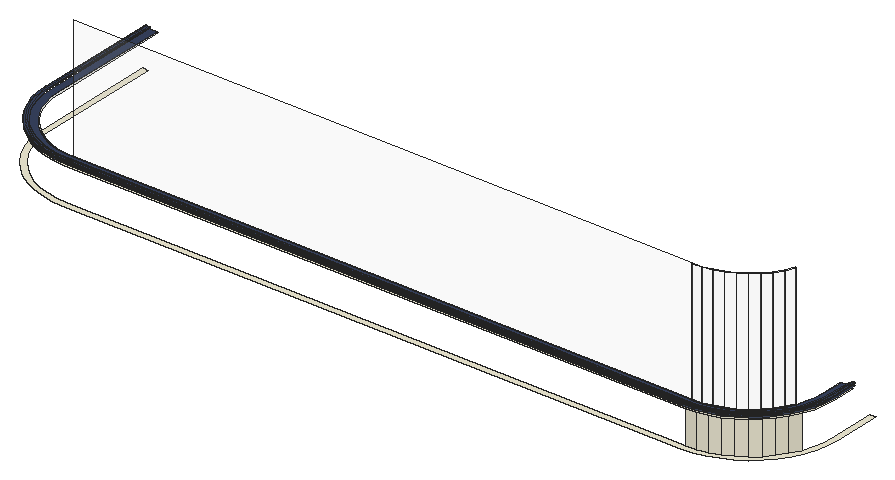
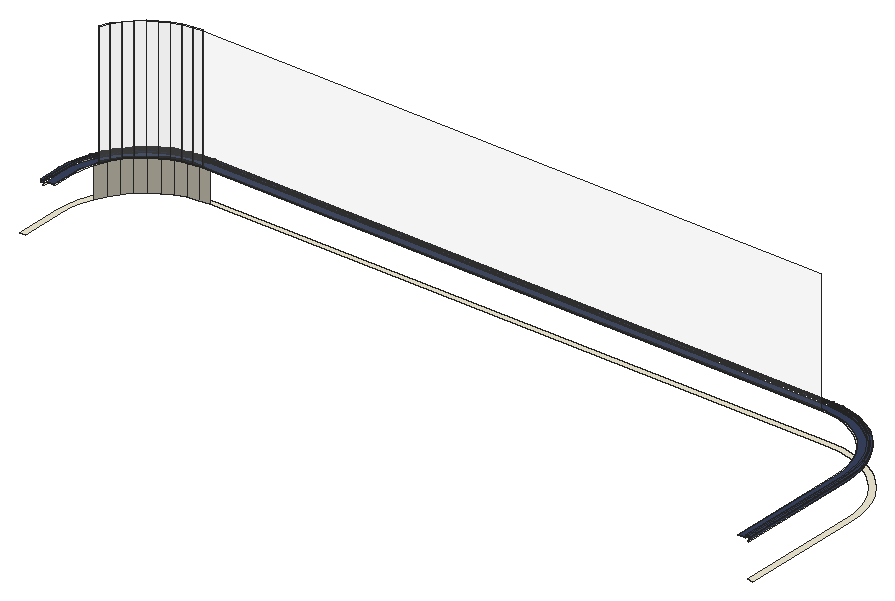
# SketchUp Ruby script. Lengths in inches.
U = 1.inch
M = Sketchup.active_model
def pt(a) = Geom::Point3d.new(a.map { |v| v * U })
def face(e, loops, mat)
  f = e.add_face(loops[0].map { |a| pt(a) })
  loops[1..].each { |l| e.add_face(l.map { |a| pt(a) }).erase! }
  f.material = f.back_material = mat if mat
  f
end
# faces: each face lists its corners as indices into pts; further lists are holes
def faces(e, pts, list, mat = nil) = list.each { |f| face(e, (f[0].is_a?(Array) ? f : [f]).map { |l| l.map { |i| pts[i] } }, mat) }
# xy, xz, yz: faces in a plane at the given z, y or x. An outline is a flat list of corners, or four numbers for a rectangle; further outlines are holes
def ring(l) = l.size == 4 ? [[l[0], l[1]], [l[2], l[1]], [l[2], l[3]], [l[0], l[3]]] : l.each_slice(2).to_a
def flat(e, list, mat, &to3) = list.each { |f| face(e, (f[0].is_a?(Array) ? f : [f]).map { |l| ring(l).map { |u, v| to3.(u, v) } }, mat) }
def xy(e, z, list, mat = nil) = flat(e, list, mat) { |x, y| [x, y, z] }
def xz(e, y, list, mat = nil) = flat(e, list, mat) { |x, z| [x, y, z] }
def yz(e, x, list, mat = nil) = flat(e, list, mat) { |y, z| [x, y, z] }
def lines(e, pts, list) = list.each { |a, b| e.add_line(pt(pts[a]), pt(pts[b])) }
# prism: a flat outline (further loops are holes) pulled along v
def prism(e, loops, v, mat = nil)
  f = face(e, loops, mat); d = Geom::Vector3d.new(v.map { |x| x * U })
  f.pushpull(f.normal.samedirection?(d) ? d.length : -d.length)
end
def box(e, o, s, mat = nil) = prism(e, [[o, [o[0] + s[0], o[1], o[2]], [o[0] + s[0], o[1] + s[1], o[2]], [o[0], o[1] + s[1], o[2]]]], [0, 0, s[2]], mat)
def at(x, y, z, deg = 0) = Geom::Transformation.translation(pt([x, y, z])) * Geom::Transformation.rotation(ORIGIN, Z_AXIS, deg.degrees)
def axes(o, x, y, z) = Geom::Transformation.new([*x, 0, *y, 0, *z, 0, *pt(o).to_a, 1])
def part(name) = M.definitions.add(name)
# library, detail: a bought-in or finely detailed component or shape, given as its bounding box
def library(name, o, s) = part(name).tap { |d| box(d.entities, o, s) }
def detail(e, o, s) = box(e.add_group.entities, o, s)
def put(e, d, t, mat = nil) = e.add_instance(d, t).tap { |i| i.material = mat if mat }
def group(e, t, mat = nil) = e.add_group.tap { |g| g.transformation = t; g.material = mat if mat }.entities
root = M.entities
M.materials.add("0344 AP 9635 Ganges Midnight-N").color = [69, 80, 105]
M.materials.add("0360 AP 9644 Monsoon Midnight-N").color = [56, 67, 95]
M.materials.add("0905 AP 7844 MILD YELLOW").color = [242, 237, 215]
M.materials.add("Glass Clear 001").color = [246, 246, 246]
M.materials["Glass Clear 001"].alpha = 0.1
xy(root,121.25,[[57,28.27,238.5625,28.27,241.91,28.49,245.21,29.14,248.39,30.22,251.4,31.71,254.19,33.57,256.71,35.79,258.93,38.31,260.79,41.1,262.28,44.11,263.36,47.29,264.01,50.59,264.23,53.9375,264.23,67.61,262.5625,67.61,262.5625,53.9375,262.36,50.8,261.74,47.73,260.74,44.75,259.35,41.9375,257.6,39.33,255.53,36.97,253.17,34.9,250.5625,33.15,247.75,31.76,244.77,30.76,241.7,30.14,238.5625,29.9375,57,29.9375,53.87,30.14,50.79,30.76,47.82,31.76,45,33.15,42.39,34.9,40.03,36.97,37.96,39.33,36.22,41.9375,34.83,44.75,33.82,47.73,33.21,50.8,33,53.9375,33,89.9375,31.33,89.9375,31.33,53.9375,31.55,50.59,32.2,47.29,33.28,44.11,34.77,41.1,36.63,38.31,38.85,35.79,41.37,33.57,44.16,31.71,47.18,30.22,50.36,29.14,53.65,28.49]],"0905 AP 7844 MILD YELLOW")
xy(root,131.3125,[[57,29.45,53.8,29.65,50.66,30.28,47.63,31.31,44.75,32.73,42.09,34.51,39.68,36.62,37.57,39.03,35.79,41.69,34.37,44.56,33.34,47.6,32.72,50.74,32.51,53.9375,32.51,89.9375,33,89.9375,33,53.9375,33.21,50.8,33.82,47.73,34.83,44.75,36.22,41.9375,37.96,39.33,40.03,36.97,42.39,34.9,45,33.15,47.82,31.76,50.79,30.76,53.87,30.14,57,29.9375,238.5625,29.9375,241.7,30.14,244.77,30.76,247.75,31.76,250.5625,33.15,253.17,34.9,255.53,36.97,257.6,39.33,259.35,41.9375,260.74,44.75,261.74,47.73,262.36,50.8,262.5625,53.9375,262.5625,60.55,263.05,60.55,263.05,53.9375,262.85,50.74,262.22,47.6,261.19,44.56,259.77,41.69,257.99,39.03,255.88,36.62,253.47,34.51,250.81,32.73,247.94,31.31,244.9,30.28,241.76,29.65,238.5625,29.45]],"0905 AP 7844 MILD YELLOW")
xy(root,132,[[57,32.3125,54.18,32.5,51.4,33.05,48.72,33.96,46.1875,35.21,43.84,36.78,41.71,38.65,39.84,40.77,38.27,43.125,37.02,45.66,36.11,48.34,35.56,51.11,35.375,53.9375,35.375,89.9375,35.75,89.9375,35.75,53.9375,35.94,51.16,36.48,48.4375,37.37,45.81,38.6,43.3125,40.14,41,41.98,38.91,44.07,37.08,46.375,35.54,48.87,34.31,51.5,33.41,54.23,32.87,57,32.69,238.5625,32.69,241.34,32.87,244.0625,33.41,246.69,34.31,249.1875,35.54,251.5,37.08,253.59,38.91,255.42,41,256.96,43.3125,258.19,45.81,259.09,48.4375,259.63,51.16,259.81,53.9375,259.81,60.0625,260.1875,60.0625,260.1875,53.9375,260,51.11,259.45,48.34,258.54,45.66,257.29,43.125,255.72,40.77,253.85,38.65,251.73,36.78,249.375,35.21,246.84,33.96,244.16,33.05,241.39,32.5,238.5625,32.3125]])
xy(root,132,[[57,29.09,53.76,29.31,50.57,29.9375,47.49,30.98,44.58,32.42,41.875,34.23,39.43,36.37,37.29,38.8125,35.48,41.51,34.05,44.43,33,47.51,32.37,50.69,32.15,53.9375,32.15,89.9375,32.51,89.9375,32.51,53.9375,32.72,50.74,33.34,47.6,34.37,44.56,35.79,41.69,37.57,39.03,39.68,36.62,42.09,34.51,44.75,32.73,47.63,31.31,50.66,30.28,53.8,29.65,57,29.45,238.5625,29.45,241.76,29.65,244.9,30.28,247.94,31.31,250.81,32.73,253.47,34.51,255.88,36.62,257.99,39.03,259.77,41.69,261.19,44.56,262.22,47.6,262.85,50.74,263.05,53.9375,263.05,60.55,262.5625,60.55,262.5625,60.91,263.41,60.91,263.41,53.9375,263.19,50.69,262.5625,47.51,261.52,44.43,260.08,41.51,258.27,38.8125,256.13,36.37,253.6875,34.23,250.99,32.42,248.07,30.98,244.99,29.9375,241.81,29.31,238.5625,29.09],[57,30.29,53.91,30.49,50.88,31.1,47.95,32.09,45.18,33.46,42.6,35.18,40.28,37.22,38.24,39.54,36.52,42.11,35.15,44.89,34.16,47.82,33.56,50.85,33.35,53.9375,33.35,89.9375,35.375,89.9375,35.375,53.9375,35.56,51.11,36.11,48.34,37.02,45.66,38.27,43.125,39.84,40.77,41.71,38.65,43.84,36.78,46.1875,35.21,48.72,33.96,51.4,33.05,54.18,32.5,57,32.3125,238.5625,32.3125,241.39,32.5,244.16,33.05,246.84,33.96,249.375,35.21,251.73,36.78,253.85,38.65,255.72,40.77,257.29,43.125,258.54,45.66,259.45,48.34,260,51.11,260.1875,53.9375,260.1875,60.0625,262.21,60.0625,262.21,53.9375,262.01,50.85,261.4,47.82,260.41,44.89,259.04,42.11,257.32,39.54,255.28,37.22,252.96,35.18,250.39,33.46,247.61,32.09,244.68,31.1,241.65,30.49,238.5625,30.29]],"0360 AP 9644 Monsoon Midnight-N")
xy(root,132.1875,[[57,30.29,238.5625,30.29,241.65,30.49,244.68,31.1,247.61,32.09,250.39,33.46,252.96,35.18,255.28,37.22,257.32,39.54,259.04,42.11,260.41,44.89,261.4,47.82,262.01,50.85,262.21,53.9375,262.21,60.0625,260.1875,60.0625,260.1875,53.9375,260,51.11,259.45,48.34,258.54,45.66,257.29,43.125,255.72,40.77,253.85,38.65,251.73,36.78,249.375,35.21,246.84,33.96,244.16,33.05,241.39,32.5,238.5625,32.3125,57,32.3125,54.18,32.5,51.4,33.05,48.72,33.96,46.1875,35.21,43.84,36.78,41.71,38.65,39.84,40.77,38.27,43.125,37.02,45.66,36.11,48.34,35.56,51.11,35.375,53.9375,35.375,89.9375,33.35,89.9375,33.35,53.9375,33.56,50.85,34.16,47.82,35.15,44.89,36.52,42.11,38.24,39.54,40.28,37.22,42.6,35.18,45.18,33.46,47.95,32.09,50.88,31.1,53.91,30.49]],"0360 AP 9644 Monsoon Midnight-N")
xy(root,132.5625,[[57,29.01,53.75,29.23,50.55,29.86,47.46,30.91,44.54,32.35,41.83,34.16,39.375,36.3125,37.23,38.76,35.41,41.47,33.97,44.4,32.92,47.49,32.29,50.68,32.07,53.9375,32.07,90.02,32.59,90.02,32.59,89.9375,32.15,89.9375,32.15,53.9375,32.37,50.69,33,47.51,34.05,44.43,35.48,41.51,37.29,38.8125,39.43,36.37,41.875,34.23,44.58,32.42,47.49,30.98,50.57,29.9375,53.76,29.31,57,29.09,238.5625,29.09,241.81,29.31,244.99,29.9375,248.07,30.98,250.99,32.42,253.6875,34.23,256.13,36.37,258.27,38.8125,260.08,41.51,261.52,44.43,262.5625,47.51,263.19,50.69,263.41,53.9375,263.41,60.91,262.5625,60.91,262.5625,60.47,262.48,60.47,262.48,60.99,263.49,60.99,263.49,53.9375,263.27,50.68,262.64,47.49,261.59,44.4,260.15,41.47,258.34,38.76,256.1875,36.3125,253.74,34.16,251.03,32.35,248.1,30.91,245.01,29.86,241.82,29.23,238.5625,29.01]],"0360 AP 9644 Monsoon Midnight-N")
xy(root,132.625,[[57,29.01,53.75,29.23,50.55,29.86,47.46,30.91,44.54,32.35,41.83,34.16,39.375,36.3125,37.23,38.76,35.41,41.47,33.97,44.4,32.92,47.49,32.29,50.68,32.07,53.9375,32.07,90.02,32.59,90.02,32.59,89.9375,32.15,89.9375,32.15,53.9375,32.37,50.69,33,47.51,34.05,44.43,35.48,41.51,37.29,38.8125,39.43,36.37,41.875,34.23,44.58,32.42,47.49,30.98,50.57,29.9375,53.76,29.31,57,29.09,238.5625,29.09,241.81,29.31,244.99,29.9375,248.07,30.98,250.99,32.42,253.6875,34.23,256.13,36.37,258.27,38.8125,260.08,41.51,261.52,44.43,262.5625,47.51,263.19,50.69,263.41,53.9375,263.41,60.91,262.5625,60.91,262.5625,60.47,262.48,60.47,262.48,60.99,263.49,60.99,263.49,53.9375,263.27,50.68,262.64,47.49,261.59,44.4,260.15,41.47,258.34,38.76,256.1875,36.3125,253.74,34.16,251.03,32.35,248.1,30.91,245.01,29.86,241.82,29.23,238.5625,29.01],[57,29.09,53.76,29.31,50.57,29.9375,47.49,30.98,44.58,32.42,41.875,34.23,39.43,36.37,37.29,38.8125,35.48,41.51,34.05,44.43,33,47.51,32.37,50.69,32.15,53.9375,32.15,89.9375,32.51,89.9375,32.51,53.9375,32.72,50.74,33.34,47.6,34.37,44.56,35.79,41.69,37.57,39.03,39.68,36.62,42.09,34.51,44.75,32.73,47.63,31.31,50.66,30.28,53.8,29.65,57,29.45,238.5625,29.45,241.76,29.65,244.9,30.28,247.94,31.31,250.81,32.73,253.47,34.51,255.88,36.62,257.99,39.03,259.77,41.69,261.19,44.56,262.22,47.6,262.85,50.74,263.05,53.9375,263.05,60.55,262.5625,60.55,262.5625,60.91,263.41,60.91,263.41,53.9375,263.19,50.69,262.5625,47.51,261.52,44.43,260.08,41.51,258.27,38.8125,256.13,36.37,253.6875,34.23,250.99,32.42,248.07,30.98,244.99,29.9375,241.81,29.31,238.5625,29.09],[57,29.45,53.8,29.65,50.66,30.28,47.63,31.31,44.75,32.73,42.09,34.51,39.68,36.62,37.57,39.03,35.79,41.69,34.37,44.56,33.34,47.6,32.72,50.74,32.51,53.9375,32.51,89.9375,32.59,89.9375,32.59,53.9375,32.8,50.75,33.42,47.62,34.45,44.6,35.86,41.73,37.63,39.08,39.74,36.68,42.14,34.57,44.79,32.8,47.66,31.38,50.68,30.36,53.8125,29.73,57,29.53,238.5625,29.53,241.75,29.73,244.88,30.36,247.9,31.38,250.77,32.8,253.42,34.57,255.82,36.68,257.93,39.08,259.7,41.73,261.12,44.6,262.14,47.62,262.77,50.75,262.97,53.9375,262.97,60.47,262.5625,60.47,262.5625,60.55,263.05,60.55,263.05,53.9375,262.85,50.74,262.22,47.6,261.19,44.56,259.77,41.69,257.99,39.03,255.88,36.62,253.47,34.51,250.81,32.73,247.94,31.31,244.9,30.28,241.76,29.65,238.5625,29.45],[57,29.53,53.8125,29.73,50.68,30.36,47.66,31.38,44.79,32.8,42.14,34.57,39.74,36.68,37.63,39.08,35.86,41.73,34.45,44.6,33.42,47.62,32.8,50.75,32.59,53.9375,32.59,89.9375,33,89.9375,33,53.9375,33.21,50.8,33.82,47.73,34.83,44.75,36.22,41.9375,37.96,39.33,40.03,36.97,42.39,34.9,45,33.15,47.82,31.76,50.79,30.76,53.87,30.14,57,29.9375,238.5625,29.9375,241.7,30.14,244.77,30.76,247.75,31.76,250.5625,33.15,253.17,34.9,255.53,36.97,257.6,39.33,259.35,41.9375,260.74,44.75,261.74,47.73,262.36,50.8,262.5625,53.9375,262.5625,60.47,262.97,60.47,262.97,53.9375,262.77,50.75,262.14,47.62,261.12,44.6,259.7,41.73,257.93,39.08,255.82,36.68,253.42,34.57,250.77,32.8,247.9,31.38,244.88,30.36,241.75,29.73,238.5625,29.53],[57,29.9375,53.87,30.14,50.79,30.76,47.82,31.76,45,33.15,42.39,34.9,40.03,36.97,37.96,39.33,36.22,41.9375,34.83,44.75,33.82,47.73,33.21,50.8,33,53.9375,33,89.9375,33.35,89.9375,33.35,53.9375,33.56,50.85,34.16,47.82,35.15,44.89,36.52,42.11,38.24,39.54,40.28,37.22,42.6,35.18,45.18,33.46,47.95,32.09,50.88,31.1,53.91,30.49,57,30.29,238.5625,30.29,241.65,30.49,244.68,31.1,247.61,32.09,250.39,33.46,252.96,35.18,255.28,37.22,257.32,39.54,259.04,42.11,260.41,44.89,261.4,47.82,262.01,50.85,262.21,53.9375,262.21,60.0625,262.5625,60.0625,262.5625,53.9375,262.36,50.8,261.74,47.73,260.74,44.75,259.35,41.9375,257.6,39.33,255.53,36.97,253.17,34.9,250.5625,33.15,247.75,31.76,244.77,30.76,241.7,30.14,238.5625,29.9375]],"0360 AP 9644 Monsoon Midnight-N")
xy(root,132.8125,[[57,29.01,238.5625,29.01,241.82,29.23,245.01,29.86,248.1,30.91,251.03,32.35,253.74,34.16,256.1875,36.3125,258.34,38.76,260.15,41.47,261.59,44.4,262.64,47.49,263.27,50.68,263.49,53.9375,263.49,60.99,262.48,60.99,262.48,60.47,262.5625,60.47,262.5625,60.91,263.41,60.91,263.41,53.9375,263.19,50.69,262.5625,47.51,261.52,44.43,260.08,41.51,258.27,38.8125,256.13,36.37,253.6875,34.23,250.99,32.42,248.07,30.98,244.99,29.9375,241.81,29.31,238.5625,29.09,57,29.09,53.76,29.31,50.57,29.9375,47.49,30.98,44.58,32.42,41.875,34.23,39.43,36.37,37.29,38.8125,35.48,41.51,34.05,44.43,33,47.51,32.37,50.69,32.15,53.9375,32.15,89.9375,32.59,89.9375,32.59,90.02,32.07,90.02,32.07,53.9375,32.29,50.68,32.92,47.49,33.97,44.4,35.41,41.47,37.23,38.76,39.375,36.3125,41.83,34.16,44.54,32.35,47.46,30.91,50.55,29.86,53.75,29.23],[57,29.09,238.5625,29.09,241.81,29.31,244.99,29.9375,248.07,30.98,250.99,32.42,253.6875,34.23,256.13,36.37,258.27,38.8125,260.08,41.51,261.52,44.43,262.5625,47.51,263.19,50.69,263.41,53.9375,263.41,60.91,262.5625,60.91,262.5625,60.55,263.05,60.55,263.05,53.9375,262.85,50.74,262.22,47.6,261.19,44.56,259.77,41.69,257.99,39.03,255.88,36.62,253.47,34.51,250.81,32.73,247.94,31.31,244.9,30.28,241.76,29.65,238.5625,29.45,57,29.45,53.8,29.65,50.66,30.28,47.63,31.31,44.75,32.73,42.09,34.51,39.68,36.62,37.57,39.03,35.79,41.69,34.37,44.56,33.34,47.6,32.72,50.74,32.51,53.9375,32.51,89.9375,32.15,89.9375,32.15,53.9375,32.37,50.69,33,47.51,34.05,44.43,35.48,41.51,37.29,38.8125,39.43,36.37,41.875,34.23,44.58,32.42,47.49,30.98,50.57,29.9375,53.76,29.31],[57,29.45,238.5625,29.45,241.76,29.65,244.9,30.28,247.94,31.31,250.81,32.73,253.47,34.51,255.88,36.62,257.99,39.03,259.77,41.69,261.19,44.56,262.22,47.6,262.85,50.74,263.05,53.9375,263.05,60.55,262.5625,60.55,262.5625,60.47,262.97,60.47,262.97,53.9375,262.77,50.75,262.14,47.62,261.12,44.6,259.7,41.73,257.93,39.08,255.82,36.68,253.42,34.57,250.77,32.8,247.9,31.38,244.88,30.36,241.75,29.73,238.5625,29.53,57,29.53,53.8125,29.73,50.68,30.36,47.66,31.38,44.79,32.8,42.14,34.57,39.74,36.68,37.63,39.08,35.86,41.73,34.45,44.6,33.42,47.62,32.8,50.75,32.59,53.9375,32.59,89.9375,32.51,89.9375,32.51,53.9375,32.72,50.74,33.34,47.6,34.37,44.56,35.79,41.69,37.57,39.03,39.68,36.62,42.09,34.51,44.75,32.73,47.63,31.31,50.66,30.28,53.8,29.65],[57,29.53,238.5625,29.53,241.75,29.73,244.88,30.36,247.9,31.38,250.77,32.8,253.42,34.57,255.82,36.68,257.93,39.08,259.7,41.73,261.12,44.6,262.14,47.62,262.77,50.75,262.97,53.9375,262.97,60.47,262.5625,60.47,262.5625,53.9375,262.36,50.8,261.74,47.73,260.74,44.75,259.35,41.9375,257.6,39.33,255.53,36.97,253.17,34.9,250.5625,33.15,247.75,31.76,244.77,30.76,241.7,30.14,238.5625,29.9375,57,29.9375,53.87,30.14,50.79,30.76,47.82,31.76,45,33.15,42.39,34.9,40.03,36.97,37.96,39.33,36.22,41.9375,34.83,44.75,33.82,47.73,33.21,50.8,33,53.9375,33,89.9375,32.59,89.9375,32.59,53.9375,32.8,50.75,33.42,47.62,34.45,44.6,35.86,41.73,37.63,39.08,39.74,36.68,42.14,34.57,44.79,32.8,47.66,31.38,50.68,30.36,53.8125,29.73],[57,29.9375,238.5625,29.9375,241.7,30.14,244.77,30.76,247.75,31.76,250.5625,33.15,253.17,34.9,255.53,36.97,257.6,39.33,259.35,41.9375,260.74,44.75,261.74,47.73,262.36,50.8,262.5625,53.9375,262.5625,60.0625,262.21,60.0625,262.21,53.9375,262.01,50.85,261.4,47.82,260.41,44.89,259.04,42.11,257.32,39.54,255.28,37.22,252.96,35.18,250.39,33.46,247.61,32.09,244.68,31.1,241.65,30.49,238.5625,30.29,57,30.29,53.91,30.49,50.88,31.1,47.95,32.09,45.18,33.46,42.6,35.18,40.28,37.22,38.24,39.54,36.52,42.11,35.15,44.89,34.16,47.82,33.56,50.85,33.35,53.9375,33.35,89.9375,33,89.9375,33,53.9375,33.21,50.8,33.82,47.73,34.83,44.75,36.22,41.9375,37.96,39.33,40.03,36.97,42.39,34.9,45,33.15,47.82,31.76,50.79,30.76,53.87,30.14]],"0360 AP 9644 Monsoon Midnight-N")
xz(root,32.69,[[57,132,238.5625,168]],"Glass Clear 001")
p = [[241.7,30.14,121.25],[241.7,30.14,131.3125],[238.5625,29.9375,131.3125],[238.5625,29.9375,121.25],[244.77,30.76,121.25],[244.77,30.76,131.3125],
  [247.75,31.76,121.25],[247.75,31.76,131.3125],[250.5625,33.15,121.25],[250.5625,33.15,131.3125],[253.17,34.9,121.25],[253.17,34.9,131.3125],
  [255.53,36.97,121.25],[255.53,36.97,131.3125],[257.6,39.33,121.25],[257.6,39.33,131.3125],[259.35,41.9375,121.25],[259.35,41.9375,131.3125],
  [260.74,44.75,121.25],[260.74,44.75,131.3125],[241.76,29.65,132],[238.5625,29.45,132],[238.5625,29.45,131.3125],[241.76,29.65,131.3125],
  [244.9,30.28,132],[244.9,30.28,131.3125],[241.7,30.14,132.625],[238.5625,29.9375,132.625],[244.77,30.76,132.625],[247.94,31.31,132],
  [247.94,31.31,131.3125],[247.75,31.76,132.625],[250.81,32.73,132],[250.81,32.73,131.3125],[250.5625,33.15,132.625],[253.47,34.51,132],
  [253.47,34.51,131.3125],[253.17,34.9,132.625],[255.88,36.62,132],[255.88,36.62,131.3125],[255.53,36.97,132.625],[257.99,39.03,132],
  [257.99,39.03,131.3125],[257.6,39.33,132.625],[259.77,41.69,132],[259.77,41.69,131.3125],[259.35,41.9375,132.625],[261.19,44.56,132],
  [261.19,44.56,131.3125],[260.74,44.75,132.625],[262.22,47.6,132],[262.22,47.6,131.3125],[238.5625,29.09,132],[241.81,29.31,132],
  [241.81,29.31,132.5625],[238.5625,29.09,132.5625],[244.99,29.9375,132],[244.99,29.9375,132.5625],[238.5625,29.45,132.625],[241.76,29.65,132.625],
  [244.9,30.28,132.625],[248.07,30.98,132],[248.07,30.98,132.5625],[241.65,30.49,132],[238.5625,30.29,132],[238.5625,30.29,132.1875],
  [241.65,30.49,132.1875],[247.94,31.31,132.625],[244.68,31.1,132],[244.68,31.1,132.1875],[250.99,32.42,132],[250.99,32.42,132.5625],
  [247.61,32.09,132],[247.61,32.09,132.1875],[250.81,32.73,132.625],[250.39,33.46,132],[250.39,33.46,132.1875],[238.5625,32.3125,132],
  [241.39,32.5,132],[241.39,32.5,132.1875],[238.5625,32.3125,132.1875],[253.6875,34.23,132],[253.6875,34.23,132.5625],[244.16,33.05,132],
  [244.16,33.05,132.1875],[241.34,32.87,132],[238.5625,32.69,132],[238.5625,32.69,168],[241.34,32.87,168],[253.47,34.51,132.625],
  [244.0625,33.41,132],[244.0625,33.41,168],[246.84,33.96,132],[246.84,33.96,132.1875],[246.69,34.31,132],[246.69,34.31,168],
  [252.96,35.18,132],[252.96,35.18,132.1875],[249.375,35.21,132],[249.375,35.21,132.1875],[256.13,36.37,132],[256.13,36.37,132.5625],
  [249.1875,35.54,132],[249.1875,35.54,168],[255.88,36.62,132.625],[251.73,36.78,132],[251.73,36.78,132.1875],[255.28,37.22,132],
  [255.28,37.22,132.1875],[251.5,37.08,132],[251.5,37.08,168],[258.27,38.8125,132],[258.27,38.8125,132.5625],[257.99,39.03,132.625],
  [253.85,38.65,132],[253.85,38.65,132.1875],[253.59,38.91,132],[253.59,38.91,168],[257.32,39.54,132],[257.32,39.54,132.1875],
  [255.72,40.77,132],[255.72,40.77,132.1875],[260.08,41.51,132],[260.08,41.51,132.5625],[255.42,41,132],[255.42,41,168],
  [259.77,41.69,132.625],[259.04,42.11,132],[259.04,42.11,132.1875],[257.29,43.125,132],[257.29,43.125,132.1875],[256.96,43.3125,132],
  [256.96,43.3125,168],[261.52,44.43,132],[261.52,44.43,132.5625],[261.19,44.56,132.625],[260.41,44.89,132],[260.41,44.89,132.1875],
  [258.54,45.66,132],[258.54,45.66,132.1875],[258.19,45.81,132],[258.19,45.81,168],[262.5625,47.51,132],[262.5625,47.51,132.5625],
  [262.22,47.6,132.625],[241.65,30.49,132.625],[238.5625,30.29,132.625],[244.68,31.1,132.625],[247.61,32.09,132.625],[250.39,33.46,132.625],
  [238.5625,32.3125,168],[241.39,32.5,168],[244.16,33.05,168],[246.84,33.96,168],[252.96,35.18,132.625],[249.375,35.21,168],
  [251.73,36.78,168],[255.28,37.22,132.625],[253.85,38.65,168],[257.32,39.54,132.625],[255.72,40.77,168],[259.04,42.11,132.625],
  [257.29,43.125,168],[260.41,44.89,132.625],[258.54,45.66,168],[238.5625,29.01,132.5625],[241.82,29.23,132.5625],[241.82,29.23,132.625],
  [238.5625,29.01,132.625],[241.82,29.23,132.8125],[238.5625,29.01,132.8125],[238.5625,29.09,132.625],[241.81,29.31,132.625],[238.5625,29.09,132.8125],
  [241.81,29.31,132.8125],[245.01,29.86,132.5625],[245.01,29.86,132.625],[245.01,29.86,132.8125],[244.99,29.9375,132.625],[244.99,29.9375,132.8125],
  [238.5625,29.45,132.8125],[241.76,29.65,132.8125],[241.75,29.73,132.625],[238.5625,29.53,132.625],[238.5625,29.53,132.8125],[241.75,29.73,132.8125],
  [244.88,30.36,132.625],[244.88,30.36,132.8125],[244.9,30.28,132.8125],[238.5625,29.9375,132.8125],[241.7,30.14,132.8125],[248.07,30.98,132.625],
  [248.07,30.98,132.8125],[248.1,30.91,132.5625],[248.1,30.91,132.625],[248.1,30.91,132.8125],[244.77,30.76,132.8125],[238.5625,30.29,132.8125],
  [241.65,30.49,132.8125],[247.94,31.31,132.8125],[247.9,31.38,132.625],[247.9,31.38,132.8125],[244.68,31.1,132.8125],[247.75,31.76,132.8125],
  [251.03,32.35,132.5625],[251.03,32.35,132.625],[251.03,32.35,132.8125],[250.99,32.42,132.625],[250.99,32.42,132.8125],[247.61,32.09,132.8125],
  [250.81,32.73,132.8125],[250.77,32.8,132.625],[250.77,32.8,132.8125],[250.5625,33.15,132.8125],[250.39,33.46,132.8125],[253.6875,34.23,132.625],
  [253.6875,34.23,132.8125],[253.74,34.16,132.5625],[253.74,34.16,132.625],[253.74,34.16,132.8125],[253.47,34.51,132.8125],[253.42,34.57,132.625],
  [253.42,34.57,132.8125],[253.17,34.9,132.8125],[252.96,35.18,132.8125],[256.13,36.37,132.625],[256.13,36.37,132.8125],[256.1875,36.3125,132.5625],
  [256.1875,36.3125,132.625],[256.1875,36.3125,132.8125],[255.88,36.62,132.8125],[255.82,36.68,132.625],[255.82,36.68,132.8125],[255.53,36.97,132.8125],
  [255.28,37.22,132.8125],[258.34,38.76,132.5625],[258.34,38.76,132.625],[258.34,38.76,132.8125],[258.27,38.8125,132.625],[258.27,38.8125,132.8125],
  [257.99,39.03,132.8125],[257.93,39.08,132.625],[257.93,39.08,132.8125],[257.6,39.33,132.8125],[257.32,39.54,132.8125],[260.08,41.51,132.625],
  [260.08,41.51,132.8125],[260.15,41.47,132.5625],[260.15,41.47,132.625],[260.15,41.47,132.8125],[259.77,41.69,132.8125],[259.7,41.73,132.625],
  [259.7,41.73,132.8125],[259.35,41.9375,132.8125],[259.04,42.11,132.8125],[261.52,44.43,132.625],[261.52,44.43,132.8125],[261.59,44.4,132.5625],
  [261.59,44.4,132.625],[261.59,44.4,132.8125],[261.12,44.6,132.625],[261.12,44.6,132.8125],[261.19,44.56,132.8125],[260.74,44.75,132.8125],
  [260.41,44.89,132.8125],[262.5625,47.51,132.625],[262.5625,47.51,132.8125],[262.64,47.49,132.5625],[262.64,47.49,132.625],[262.64,47.49,132.8125],
  [262.22,47.6,132.8125]]
faces(root,p,[[0,1,2,3],[4,5,1,0],[6,7,5,4],[8,9,7,6],[10,11,9,8],[12,13,11,10],[14,15,13,12],[16,17,15,14],
  [18,19,17,16],[20,21,22,23],[24,20,23,25],[29,24,25,30],[32,29,30,33],[35,32,33,36],[38,35,36,39],[41,38,39,42],
  [44,41,42,45],[47,44,45,48],[50,47,48,51]],"0905 AP 7844 MILD YELLOW")
faces(root,p,[[1,26,27,2],[5,28,26,1],[7,31,28,5],[9,34,31,7],[11,37,34,9],[13,40,37,11],[15,43,40,13],[17,46,43,15],
  [19,49,46,17],[20,21,58,59],[24,20,59,60],[29,24,60,67],[32,29,67,74],[35,32,74,89],[38,35,89,104],[41,38,104,113],
  [44,41,113,126],[47,44,126,135],[50,47,135,144],[54,55,171,172],[57,54,172,178],[62,57,178,191],[71,62,191,207],[82,71,207,215],
  [101,82,215,225],[112,101,225,238],[123,112,238,245],[134,123,245,255],[143,134,255,265]])
faces(root,p,[[52,53,54,55],[53,56,57,54],[56,61,62,57],[61,70,71,62],[70,81,82,71],[81,100,101,82],[100,111,112,101],[111,122,123,112],
  [122,133,134,123],[133,142,143,134]],"0344 AP 9635 Ganges Midnight-N")
faces(root,p,[[63,64,65,66],[68,63,66,69],[72,68,69,73],[75,72,73,76],[77,78,79,80],[78,83,84,79],[83,92,93,84],[96,75,76,97],
  [92,98,99,93],[98,105,106,99],[107,96,97,108],[105,114,115,106],[118,107,108,119],[114,120,121,115],[127,118,119,128],[120,129,130,121],
  [136,127,128,137],[129,138,139,130],[145,66,65,146],[147,69,66,145],[148,73,69,147],[149,76,73,148],[154,97,76,149],[157,108,97,154],
  [159,119,108,157],[161,128,119,159],[163,137,128,161],[165,166,167,168],[168,167,169,170],[172,171,173,174],[166,175,176,167],[167,176,177,169],
  [178,172,174,179],[59,58,180,181],[182,183,184,185],[186,182,185,187],[60,59,181,188],[26,27,189,190],[191,178,179,192],[175,193,194,176],
  [176,194,195,177],[28,26,190,196],[145,146,197,198],[67,60,188,199],[200,186,187,201],[147,145,198,202],[31,28,196,203],[193,204,205,194],
  [194,205,206,195],[207,191,192,208],[148,147,202,209],[74,67,199,210],[211,200,201,212],[34,31,203,213],[149,148,209,214],[215,207,208,216],
  [204,217,218,205],[205,218,219,206],[89,74,210,220],[221,211,212,222],[37,34,213,223],[154,149,214,224],[225,215,216,226],[217,227,228,218],
  [218,228,229,219],[104,89,220,230],[231,221,222,232],[40,37,223,233],[157,154,224,234],[227,235,236,228],[228,236,237,229],[238,225,226,239],
  [113,104,230,240],[241,231,232,242],[43,40,233,243],[159,157,234,244],[245,238,239,246],[235,247,248,236],[236,248,249,237],[126,113,240,250],
  [251,241,242,252],[46,43,243,253],[161,159,244,254],[255,245,246,256],[247,257,258,248],[248,258,259,249],[260,251,252,261],[135,126,250,262],
  [49,46,253,263],[163,161,254,264],[265,255,256,266],[257,267,268,258],[258,268,269,259],[144,135,262,270]],"0360 AP 9644 Monsoon Midnight-N")
faces(root,p,[[85,86,87,88],[90,85,88,91],[94,90,91,95],[102,94,95,103],[109,102,103,110],[116,109,110,117],[124,116,117,125],[131,124,125,132],
  [140,131,132,141],[150,80,79,151],[151,79,84,152],[152,84,93,153],[153,93,99,155],[155,99,106,156],[156,106,115,158],[158,115,121,160],
  [160,121,130,162],[162,130,139,164]],"Glass Clear 001")
